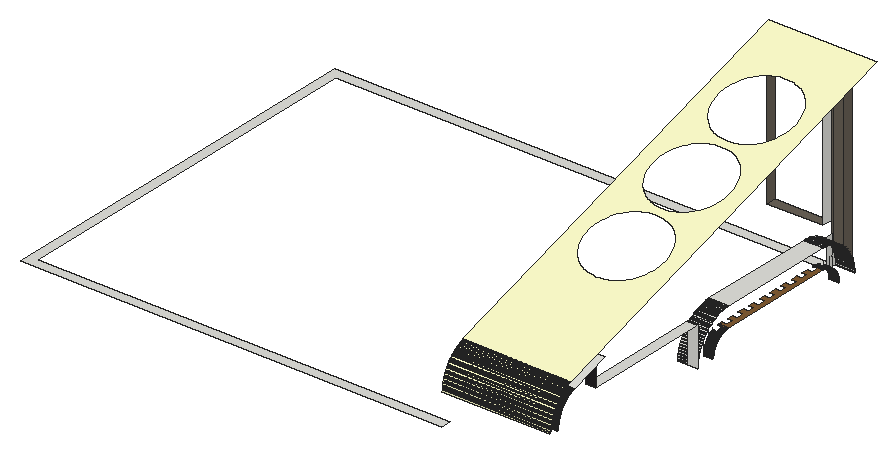
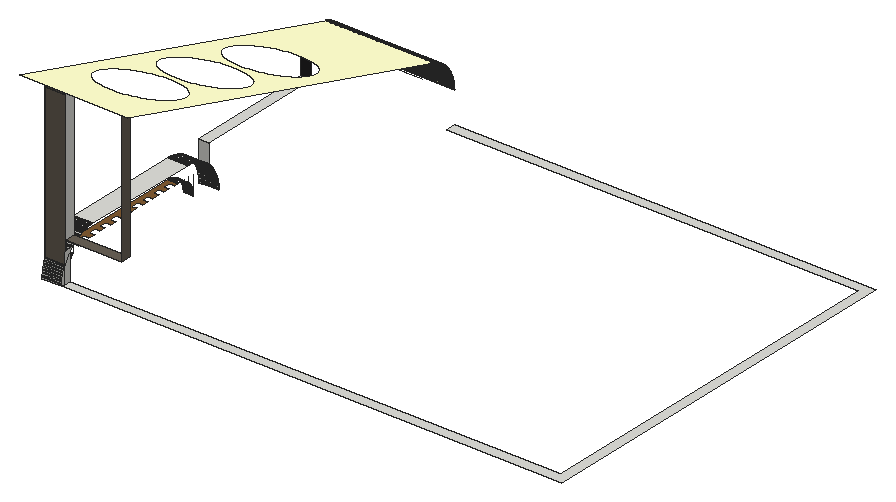
# SketchUp Ruby script. Lengths in inches.
U = 1.inch
M = Sketchup.active_model
def pt(a) = Geom::Point3d.new(a.map { |v| v * U })
def face(e, loops, mat)
  f = e.add_face(loops[0].map { |a| pt(a) })
  loops[1..].each { |l| e.add_face(l.map { |a| pt(a) }).erase! }
  f.material = f.back_material = mat if mat
  f
end
# faces: each face lists its corners as indices into pts; further lists are holes
def faces(e, pts, list, mat = nil) = list.each { |f| face(e, (f[0].is_a?(Array) ? f : [f]).map { |l| l.map { |i| pts[i] } }, mat) }
# xy, xz, yz: faces in a plane at the given z, y or x. An outline is a flat list of corners, or four numbers for a rectangle; further outlines are holes
def ring(l) = l.size == 4 ? [[l[0], l[1]], [l[2], l[1]], [l[2], l[3]], [l[0], l[3]]] : l.each_slice(2).to_a
def flat(e, list, mat, &to3) = list.each { |f| face(e, (f[0].is_a?(Array) ? f : [f]).map { |l| ring(l).map { |u, v| to3.(u, v) } }, mat) }
def xy(e, z, list, mat = nil) = flat(e, list, mat) { |x, y| [x, y, z] }
def xz(e, y, list, mat = nil) = flat(e, list, mat) { |x, z| [x, y, z] }
def yz(e, x, list, mat = nil) = flat(e, list, mat) { |y, z| [x, y, z] }
def lines(e, pts, list) = list.each { |a, b| e.add_line(pt(pts[a]), pt(pts[b])) }
# prism: a flat outline (further loops are holes) pulled along v
def prism(e, loops, v, mat = nil)
  f = face(e, loops, mat); d = Geom::Vector3d.new(v.map { |x| x * U })
  f.pushpull(f.normal.samedirection?(d) ? d.length : -d.length)
end
def box(e, o, s, mat = nil) = prism(e, [[o, [o[0] + s[0], o[1], o[2]], [o[0] + s[0], o[1] + s[1], o[2]], [o[0], o[1] + s[1], o[2]]]], [0, 0, s[2]], mat)
def at(x, y, z, deg = 0) = Geom::Transformation.translation(pt([x, y, z])) * Geom::Transformation.rotation(ORIGIN, Z_AXIS, deg.degrees)
def axes(o, x, y, z) = Geom::Transformation.new([*x, 0, *y, 0, *z, 0, *pt(o).to_a, 1])
def part(name) = M.definitions.add(name)
# library, detail: a bought-in or finely detailed component or shape, given as its bounding box
def library(name, o, s) = part(name).tap { |d| box(d.entities, o, s) }
def detail(e, o, s) = box(e.add_group.entities, o, s)
def put(e, d, t, mat = nil) = e.add_instance(d, t).tap { |i| i.material = mat if mat }
def group(e, t, mat = nil) = e.add_group.tap { |g| g.transformation = t; g.material = mat if mat }.entities
root = M.entities
M.materials.add("C08_Toffee_Ember").color = [130, 92, 50]
M.materials.add("E01_Mint_Frost").color = [255, 255, 204]
M.materials.add("Marble_07_1K").color = [36, 34, 36]
M.materials.add("Plaster_04_1K").color = [106, 98, 87]
xy(root,396,[[5.5,15,263.5,15,263.5,21,11.5,21,11.5,249,311.5,249,311.5,255,5.5,255]])
xy(root,408,[[317.5,159,317.5,161.32,320.5,161.32,320.5,165.4,317.5,165.4,317.5,169.49,320.5,169.49,320.5,173.57,317.5,173.57,317.5,177.66,320.5,177.66,320.5,181.74,317.5,181.74,317.5,185.82,320.5,185.82,320.5,189.91,317.5,189.91,317.5,193.99,320.5,193.99,320.5,198.08,317.5,198.08,317.5,202.16,320.5,202.16,320.5,206.24,317.5,206.24,317.5,210.33,320.5,210.33,320.5,214.41,317.5,214.41,317.5,218.5,320.5,218.5,320.5,222.58,317.5,222.58,317.5,226.66,320.5,226.66,320.5,230.75,317.5,230.75,317.5,231,323.5,231,323.5,159],[317.5,231,323.5,231.38]],"C08_Toffee_Ember")
xy(root,420,[[317.5,57,323.5,135],[311.5,159,323.5,231]])
xy(root,421,[[276.5,247,310.5,253]],"Plaster_04_1K")
xz(root,20.99,[[323.5,414.47,329.5,414.95]])
xz(root,57,[[317.5,420,323.5,437.47]],"Marble_07_1K")
xz(root,135,[[317.5,396,323.5,420]])
xz(root,243,[[317.5,396,323.5,396.38]],"C08_Toffee_Ember")
xz(root,247,[[317.5,413.98,323.5,498]],"Plaster_04_1K")
xz(root,253,[[311.5,406.93,323.5,500.01]],"Plaster_04_1K")
yz(root,276.5,[[247,421,253,503]],"Plaster_04_1K")
yz(root,310.5,[[247,421,253,503]])
yz(root,311.5,[[249,396,249,411.97,249.05,411.92,249.54,411.34,250.01,410.75,250.47,410.15,250.9,409.53,251.3125,408.9,251.71,408.25,251.85,408,252.08,407.6,252.43,406.93,252.76,406.25,253,405.72,253,396],[253,396,253,405.72,253.07,405.56,253.36,404.86,253.62,404.15,253.86,403.4375,254.08,402.71,254.28,401.98,254.45,401.25,254.6,400.51,254.73,399.76,254.83,399.01,254.91,398.26,254.96,397.51,254.99,396.76,255,396],[253,405.72,253,413.98,247,413.98,247.48,413.54,248.02,413.02,248.54,412.48,249,411.97,249.05,411.92,249.54,411.34,250.01,410.75,250.47,410.15,250.9,409.53,251.3125,408.9,251.71,408.25,251.85,408,252.08,407.6,252.43,406.93,252.76,406.25]])
yz(root,323.5,[[21,414,21,415.2,20.99,414.95,20.99,414.47]])
yz(root,323.5,[[252.43,406.93,253,406.93,253,500.01,247,498.15,247,413.98,247.48,413.54,248.02,413.02,248.54,412.48,249.05,411.92,249.54,411.34,250.01,410.75,250.47,410.15,250.9,409.53,251.3125,408.9,251.71,408.25,251.85,408,252.08,407.6]],"Plaster_04_1K")
p = [[317.5,135,396],[323.5,135,396],[323.5,135.03,396.75],[311.5,135.03,396.75],[311.5,135,396],[317.5,147,396],
  [317.5,147.01,396.375],[323.5,147.01,396.375],[323.5,147,396],[311.5,254.99,396.76],[323.5,254.99,396.76],[323.5,255,396],
  [311.5,255,396],[317.5,147.03,396.75],[323.5,147.03,396.75],[317.5,242.98,396.76],[317.5,243,396.38],[323.5,243,396.38],
  [323.5,242.98,396.76],[323.5,135.08,397.5],[311.5,135.08,397.5],[317.5,147.07,397.125],[323.5,147.07,397.125],[317.5,242.96,397.13],
  [323.5,242.96,397.13],[311.5,254.96,397.51],[323.5,254.96,397.51],[317.5,147.11,397.5],[323.5,147.11,397.5],[317.5,242.92,397.51],
  [323.5,242.92,397.51],[323.5,135.15,398.24],[311.5,135.15,398.24],[317.5,147.17,397.87],[323.5,147.17,397.87],[317.5,242.87,397.88],
  [323.5,242.87,397.88],[311.5,254.91,398.26],[323.5,254.91,398.26],[317.5,147.24,398.24],[323.5,147.24,398.24],[317.5,242.81,398.26],
  [323.5,242.81,398.26],[323.5,135.24,398.99],[311.5,135.24,398.99],[317.5,147.32,398.61],[323.5,147.32,398.61],[317.5,242.74,398.63],
  [323.5,242.74,398.63],[311.5,254.83,399.01],[323.5,254.83,399.01],[317.5,147.41,398.97],[323.5,147.41,398.97],[317.5,242.65,399],
  [323.5,242.65,399],[323.5,135.36,399.73],[311.5,135.36,399.73],[317.5,147.51,399.33],[323.5,147.51,399.33],[317.5,242.55,399.36],
  [323.5,242.55,399.36],[311.5,254.73,399.76],[323.5,254.73,399.76],[317.5,147.625,399.6875],[323.5,147.625,399.6875],[317.5,242.45,399.72],
  [323.5,242.45,399.72],[323.5,135.5,400.47],[311.5,135.5,400.47],[317.5,147.75,400.04],[323.5,147.75,400.04],[317.5,242.33,400.08],
  [323.5,242.33,400.08],[311.5,254.6,400.51],[323.5,254.6,400.51],[317.5,147.88,400.39],[323.5,147.88,400.39],[317.5,242.19,400.4375],
  [323.5,242.19,400.4375],[317.5,148.03,400.74],[323.5,148.03,400.74],[317.5,242.05,400.79],[323.5,242.05,400.79],[323.5,135.66,401.2],
  [311.5,135.66,401.2],[311.5,254.45,401.25],[323.5,254.45,401.25],[317.5,148.1875,401.08],[323.5,148.1875,401.08],[317.5,241.9,401.13],
  [323.5,241.9,401.13],[317.5,148.35,401.42],[323.5,148.35,401.42],[317.5,241.73,401.47],[323.5,241.73,401.47],[323.5,135.85,401.92],
  [311.5,135.85,401.92],[311.5,254.28,401.98],[323.5,254.28,401.98],[317.5,148.53,401.75],[323.5,148.53,401.75],[317.5,241.56,401.81],
  [323.5,241.56,401.81],[317.5,148.72,402.07],[323.5,148.72,402.07],[317.5,241.37,402.14],[323.5,241.37,402.14],[323.5,136.06,402.65],
  [311.5,136.06,402.65],[311.5,254.08,402.71],[323.5,254.08,402.71],[317.5,148.92,402.39],[323.5,148.92,402.39],[317.5,241.17,402.46],
  [323.5,241.17,402.46],[317.5,149.12,402.71],[323.5,149.12,402.71],[317.5,240.97,402.78],[323.5,240.97,402.78],[323.5,136.29,403.36],
  [311.5,136.29,403.36],[317.5,149.34,403.01],[323.5,149.34,403.01],[311.5,253.86,403.4375],[323.5,253.86,403.4375],[317.5,240.75,403.09],
  [323.5,240.75,403.09],[317.5,149.57,403.3125],[323.5,149.57,403.3125],[317.5,240.52,403.39],[323.5,240.52,403.39],[317.5,149.8,403.61],
  [323.5,149.8,403.61],[323.5,136.54,404.07],[311.5,136.54,404.07],[317.5,240.29,403.6875],[323.5,240.29,403.6875],[311.5,253.62,404.15],
  [323.5,253.62,404.15],[317.5,150.05,403.89],[323.5,150.05,403.89],[317.5,240.04,403.97],[323.5,240.04,403.97],[317.5,150.3,404.17],
  [323.5,150.3,404.17],[317.5,239.79,404.25],[323.5,239.79,404.25],[323.5,136.81,404.76],[311.5,136.81,404.76],[317.5,150.56,404.44],
  [323.5,150.56,404.44],[311.5,253.36,404.86],[323.5,253.36,404.86],[317.5,239.53,404.53],[323.5,239.53,404.53],[317.5,150.58,404.46],
  [317.5,150.83,404.7],[323.5,150.83,404.7],[317.5,239.25,404.79],[323.5,239.25,404.79],[317.5,151.11,404.95],[323.5,151.11,404.95],
  [323.5,137.1,405.45],[311.5,137.1,405.45],[317.5,238.97,405.04],[323.5,238.97,405.04],[311.5,253.07,405.56],[323.5,253.07,405.56],
  [317.5,151.39,405.2],[323.5,151.39,405.2],[323.5,238.6875,405.29],[320.5,238.6875,405.29],[320.5,238.92,405.09],[317.5,238.92,405.09],
  [317.5,151.6875,405.43],[323.5,151.6875,405.43],[323.5,238.39,405.52],[320.5,238.39,405.52],[317.5,151.99,405.66],[323.5,151.99,405.66],
  [323.5,137.42,406.14],[311.5,137.42,406.14],[323.5,238.09,405.75],[320.5,238.09,405.75],[311.5,252.76,406.25],[323.5,252.76,406.25],
  [311.5,253,405.72],[317.5,152.29,405.88],[323.5,152.29,405.88],[323.5,237.78,405.97],[320.5,237.78,405.97],[317.5,152.61,406.08],
  [323.5,152.61,406.08],[323.5,237.46,406.17],[320.5,237.46,406.17],[323.5,137.75,406.81],[311.5,137.75,406.81],[317.5,152.93,406.28],
  [323.5,152.93,406.28],[323.5,237.14,406.37],[320.5,237.14,406.37],[311.5,252.43,406.93],[323.5,252.43,406.93],[317.5,153.25,406.47],
  [323.5,153.25,406.47],[323.5,236.81,406.56],[320.5,236.81,406.56],[317.5,153.58,406.65],[323.5,153.58,406.65],[317.5,153.92,406.8125],
  [323.5,153.92,406.8125],[323.5,236.47,406.73],[320.5,236.47,406.73],[323.5,236.13,406.9],[320.5,236.13,406.9],[323.5,138.11,407.47],
  [311.5,138.11,407.47],[317.5,154.16,406.92],[320.5,154.16,406.92],[320.5,154.26,406.97],[323.5,154.26,406.97],[323.5,235.79,407.05],
  [320.5,235.79,407.05],[311.5,252.08,407.6],[323.5,252.08,407.6],[320.5,154.61,407.12],[323.5,154.61,407.12],[320.5,154.96,407.25],
  [323.5,154.96,407.25],[323.5,235.4375,407.19],[320.5,235.4375,407.19],[323.5,235.08,407.33],[320.5,235.08,407.33],[320.5,155.3125,407.375],
  [323.5,155.3125,407.375],[317.5,234.72,407.45],[317.5,234.83,407.41],[320.5,234.83,407.41],[323.5,234.72,407.45],[320.5,155.67,407.49],
  [323.5,155.67,407.49],[317.5,234.36,407.55],[323.5,234.36,407.55],[323.5,138.48,408.11],[311.5,138.48,408.11],[320.5,156.03,407.59],
  [323.5,156.03,407.59],[320.5,156.39,407.68],[323.5,156.39,407.68],[317.5,234,407.65],[323.5,234,407.65],[311.5,251.85,408],
  [323.5,251.85,408],[320.5,156.76,407.76],[323.5,156.76,407.76],[317.5,233.26,407.81],[317.5,233.63,407.74],[323.5,233.63,407.74],
  [323.5,233.26,407.81],[320.5,157.13,407.83],[323.5,157.13,407.83],[320.5,157.5,407.89],[323.5,157.5,407.89],[317.5,232.88,407.87],
  [323.5,232.88,407.87],[320.5,157.74,407.92],[317.5,157.74,407.92],[317.5,157.875,407.93],[323.5,157.875,407.93],[317.5,158.25,407.97],
  [323.5,158.25,407.97],[317.5,232.13,407.96],[317.5,232.51,407.92],[323.5,232.51,407.92],[323.5,232.13,407.96],[317.5,158.625,407.99],
  [323.5,158.625,407.99],[317.5,159,408],[323.5,159,408],[317.5,231.38,408],[317.5,231.76,407.98],[323.5,231.76,407.98],
  [323.5,231.38,408],[311.5,251.71,408.25],[323.5,251.71,408.25],[323.5,138.88,408.75],[311.5,138.88,408.75],[311.5,251.3125,408.9],
  [323.5,251.3125,408.9],[323.5,139.3,409.375],[311.5,139.3,409.375],[311.5,250.9,409.53],[323.5,250.9,409.53],[323.5,139.73,409.99],
  [311.5,139.73,409.99],[311.5,250.47,410.15],[323.5,250.47,410.15],[323.5,140.18,410.59],[311.5,140.18,410.59],[311.5,250.01,410.75],
  [323.5,250.01,410.75],[323.5,140.65,411.17],[311.5,140.65,411.17],[311.5,249.54,411.34],[323.5,249.54,411.34],[323.5,141.14,411.74],
  [311.5,141.14,411.74],[311.5,141,411.58],[311.5,249.05,411.92],[323.5,249.05,411.92],[323.5,141.65,412.29],[311.5,141.65,412.29],
  [311.5,248.54,412.48],[323.5,248.54,412.48],[311.5,249,411.97],[323.5,142.17,412.83],[311.5,142.17,412.83],[311.5,248.02,413.02],
  [323.5,248.02,413.02],[323.5,142.71,413.35],[311.5,142.71,413.35],[311.5,247.48,413.54],[323.5,247.48,413.54],[323.5,143.26,413.86],
  [311.5,143.26,413.86],[311.5,247,413.98],[317.5,247,413.98],[323.5,247,413.98],[323.5,143.83,414.35],[311.5,143.83,414.35],
  [323.5,21,414],[323.5,20.99,414.47],[329.5,20.99,414.47],[329.5,21,414],[323.5,246.92,414.05],[311.5,246.92,414.05],
  [311.5,246.34,414.54],[323.5,246.34,414.54],[323.5,144.41,414.82],[311.5,144.41,414.82],[311.5,245.75,415.01],[323.5,245.75,415.01],
  [323.5,145.01,415.27],[311.5,145.01,415.27],[323.5,20.99,414.95],[323.5,21,415.2],[329.5,21,415.2],[329.5,20.99,414.95],
  [311.5,245.15,415.47],[323.5,245.15,415.47],[323.5,21.01,415.42],[329.5,21.01,415.42],[263.5,15,415.29],[329.5,15,415.29],
  [329.5,15.02,415.87],[263.5,15.02,415.87],[323.5,145.625,415.7],[311.5,145.625,415.7],[323.5,21.03,415.9],[329.5,21.03,415.9],
  [311.5,244.53,415.9],[323.5,244.53,415.9],[323.5,146.25,416.12],[311.5,146.25,416.12],[329.5,15.0625,416.5],[263.5,15.0625,416.5],
  [323.5,21.07,416.37],[329.5,21.07,416.37],[311.5,243.9,416.3125],[323.5,243.9,416.3125],[323.5,146.89,416.52],[311.5,146.89,416.52],
  [311.5,243.25,416.71],[323.5,243.25,416.71],[323.5,21.125,416.84],[329.5,21.125,416.84],[329.5,15.12,417.12],[263.5,15.12,417.12],
  [323.5,147.53,416.89],[311.5,147.53,416.89],[311.5,242.6,417.08],[323.5,242.6,417.08],[323.5,21.19,417.31],[329.5,21.19,417.31],
  [323.5,148.19,417.25],[311.5,148.19,417.25],[329.5,15.19,417.74],[263.5,15.19,417.74],[311.5,241.93,417.43],[323.5,241.93,417.43],
  [323.5,148.86,417.58],[311.5,148.86,417.58],[323.5,21.27,417.78],[329.5,21.27,417.78],[311.5,241.25,417.76],[323.5,241.25,417.76],
  [323.5,149.55,417.9],[311.5,149.55,417.9],[329.5,15.28,418.36],[263.5,15.28,418.36],[323.5,21.36,418.24],[329.5,21.36,418.24],
  [311.5,240.56,418.07],[323.5,240.56,418.07],[323.5,150.24,418.19],[311.5,150.24,418.19],[311.5,239.86,418.36],[323.5,239.86,418.36],
  [323.5,21.46,418.71],[329.5,21.46,418.71],[323.5,150.93,418.46],[311.5,150.93,418.46],[329.5,15.39,418.97],[263.5,15.39,418.97],
  [311.5,239.15,418.62],[323.5,239.15,418.62],[311.5,239.59,418.46],[323.5,151.64,418.71],[311.5,151.64,418.71],[311.5,238.4375,418.86],
  [323.5,238.4375,418.86],[323.5,21.57,419.17],[329.5,21.57,419.17],[323.5,152.35,418.94],[311.5,152.35,418.94],[323.5,153.08,419.15],
  [311.5,153.08,419.15],[311.5,237.71,419.08],[323.5,237.71,419.08],[329.5,15.51,419.58],[263.5,15.51,419.58],[311.5,236.98,419.28],
  [323.5,236.98,419.28],[323.5,21.7,419.625],[329.5,21.7,419.625],[323.5,153.8,419.34],[311.5,153.8,419.34],[323.5,154.53,419.5],
  [311.5,154.53,419.5],[311.5,236.25,419.45],[323.5,236.25,419.45],[323.5,155.27,419.64],[311.5,155.27,419.64],[311.5,235.51,419.6],
  [323.5,235.51,419.6],[329.5,15.65,420.19],[263.5,15.65,420.19],[323.5,21.84,420.08],[329.5,21.84,420.08],[323.5,156.01,419.76],
  [311.5,156.01,419.76],[311.5,234.76,419.73],[323.5,234.76,419.73],[311.5,234.01,419.83],[323.5,234.01,419.83],[323.5,156.76,419.85],
  [311.5,156.76,419.85],[311.5,233.26,419.91],[323.5,233.26,419.91],[323.5,157.5,419.92],[311.5,157.5,419.92],[323.5,158.25,419.97],
  [311.5,158.25,419.97],[311.5,232.51,419.96],[323.5,232.51,419.96],[323.5,159,420],[311.5,159,420],[311.5,231,420],
  [323.5,231,420],[323.5,231.76,419.99],[311.5,231.76,419.99],[323.5,21.99,420.53],[329.5,21.99,420.53],[329.5,15.81,420.8],
  [263.5,15.81,420.8],[323.5,22.15,420.97],[329.5,22.15,420.97],[329.5,15.98,421.4],[263.5,15.98,421.4],[323.5,22.32,421.41],
  [329.5,22.32,421.41],[329.5,16.16,421.99],[263.5,16.16,421.99],[323.5,22.51,421.85],[329.5,22.51,421.85],[323.5,22.7,422.28],
  [329.5,22.7,422.28],[329.5,16.37,422.58],[263.5,16.37,422.58],[323.5,22.91,422.71],[329.5,22.91,422.71],[329.5,16.58,423.17],
  [263.5,16.58,423.17],[323.5,23.13,423.13],[329.5,23.13,423.13],[323.5,23.36,423.54],[329.5,23.36,423.54],[329.5,16.82,423.75],
  [263.5,16.82,423.75],[323.5,23.6,423.95],[329.5,23.6,423.95],[329.5,17.07,424.32],[263.5,17.07,424.32],[323.5,23.85,424.35],
  [329.5,23.85,424.35],[329.5,17.33,424.89],[263.5,17.33,424.89],[323.5,24.11,424.75],[329.5,24.11,424.75],[323.5,24.39,425.14],
  [329.5,24.39,425.14],[329.5,17.61,425.44],[263.5,17.61,425.44],[323.5,24.67,425.52],[329.5,24.67,425.52],[329.5,17.9,426],
  [263.5,17.9,426],[323.5,24.96,425.89],[329.5,24.96,425.89],[323.5,25.26,426.26],[329.5,25.26,426.26],[329.5,18.21,426.54],
  [263.5,18.21,426.54],[323.5,25.58,426.61],[329.5,25.58,426.61],[329.5,18.53,427.07],[263.5,18.53,427.07],[323.5,25.9,426.96],
  [329.5,25.9,426.96],[323.5,26.23,427.3],[329.5,26.23,427.3],[329.5,18.87,427.6],[263.5,18.87,427.6],[323.5,26.57,427.64],
  [329.5,26.57,427.64],[329.5,19.22,428.12],[263.5,19.22,428.12],[323.5,26.91,427.96],[329.5,26.91,427.96],[323.5,27.27,428.27],
  [329.5,27.27,428.27],[329.5,19.58,428.625],[263.5,19.58,428.625],[323.5,27.63,428.58],[329.5,27.63,428.58],[329.5,19.96,429.12],
  [263.5,19.96,429.12],[323.5,28.01,428.87],[329.5,28.01,428.87],[323.5,28.39,429.15],[329.5,28.39,429.15],[329.5,20.35,429.61],
  [263.5,20.35,429.61],[323.5,28.77,429.43],[329.5,28.77,429.43],[323.5,29.17,429.69],[329.5,29.17,429.69],[329.5,20.75,430.09],
  [263.5,20.75,430.09],[323.5,29.57,429.94],[329.5,29.57,429.94],[323.5,29.98,430.1875],[329.5,29.98,430.1875],[329.5,21.17,430.55],
  [263.5,21.17,430.55],[263.5,21,430.37],[323.5,30.39,430.42],[329.5,30.39,430.42],[323.5,30.81,430.64],[329.5,30.81,430.64],
  [329.5,21.59,431.01],[263.5,21.59,431.01],[323.5,31.23,430.85],[329.5,31.23,430.85],[323.5,31.67,431.05],[329.5,31.67,431.05],
  [329.5,22.03,431.45],[263.5,22.03,431.45],[323.5,32.1,431.23],[329.5,32.1,431.23],[323.5,32.54,431.41],[329.5,32.54,431.41],
  [323.5,32.99,431.57],[329.5,32.99,431.57],[329.5,22.49,431.88],[263.5,22.49,431.88],[323.5,33.4375,431.72],[329.5,33.4375,431.72],
  [323.5,57,439.04],[329.5,57,439.04],[323.5,38,433.14],[323.5,39,433.45],[323.5,40,433.76],[329.5,22.95,432.3],
  [263.5,22.95,432.3],[263.5,22.61,432],[329.5,23.42,432.71],[263.5,23.42,432.71],[329.5,23.9,433.1],[263.5,23.9,433.1],
  [329.5,24.4,433.49],[263.5,24.4,433.49],[329.5,24.9,433.85],[263.5,24.9,433.85],[329.5,25.42,434.21],[263.5,25.42,434.21],
  [329.5,25.9375,434.55],[263.5,25.9375,434.55],[329.5,26.47,434.88],[263.5,26.47,434.88],[329.5,27.01,435.19],[263.5,27.01,435.19],
  [329.5,27.56,435.49],[263.5,27.56,435.49],[329.5,28.12,435.77],[263.5,28.12,435.77],[329.5,28.68,436.04],[263.5,28.68,436.04],
  [329.5,29.25,436.3],[263.5,29.25,436.3],[329.5,29.83,436.54],[263.5,29.83,436.54],[329.5,30.41,436.76],[263.5,30.41,436.76],
  [329.5,30.96,436.95],[263.5,30.96,436.95],[329.5,264.19,509.34],[263.5,264.19,509.34],[263.5,247,504],[294.99,137.32,469.96],
  [296.5,137.37,469.98],[298.01,137.32,469.96],[299.51,137.1875,469.92],[301,136.96,469.85],[302.47,136.65,469.75],[303.92,136.24,469.63],
  [305.33,135.76,469.48],[306.72,135.18,469.3],[308.0625,134.53,469.1],[309.36,133.8,468.87],[310.61,132.99,468.62],[311.8,132.11,468.34],
  [312.93,131.15,468.05],[314,130.14,467.73],[314.99,129.06,467.4],[315.92,127.92,467.04],[316.76,126.73,466.67],[317.53,125.49,466.29],
  [318.22,124.2,465.89],[318.81,122.88,465.48],[319.33,121.53,465.06],[319.75,120.15,464.63],[320.07,118.74,464.2],[320.3125,117.32,463.75],
  [320.45,115.88,463.31],[320.5,114.44,462.86],[320.45,113.01,462.42],[320.3125,111.57,461.97],[320.07,110.15,461.53],[319.75,108.74,461.09],
  [319.33,107.36,460.66],[318.81,106.01,460.24],[318.22,104.69,459.83],[317.53,103.4,459.44],[316.76,102.16,459.05],[315.92,100.97,458.68],
  [314.99,99.83,458.33],[314,98.75,457.99],[312.93,97.74,457.68],[311.8,96.78,457.38],[310.61,95.9,457.11],[309.36,95.09,456.86],
  [308.0625,94.36,456.63],[306.72,93.7,456.43],[305.33,93.13,456.25],[303.92,92.65,456.1],[302.47,92.24,455.97],[301,91.93,455.875],
  [299.51,91.7,455.8],[298.01,91.57,455.76],[297.99,91.57,455.76],[296.5,91.52,455.75],[295.01,91.57,455.76],[294.99,91.57,455.76],
  [293.49,91.7,455.8],[292,91.93,455.875],[290.53,92.24,455.97],[289.08,92.65,456.1],[287.67,93.13,456.25],[286.28,93.7,456.43],
  [284.9375,94.36,456.63],[283.64,95.09,456.86],[282.39,95.9,457.11],[281.2,96.78,457.38],[280.07,97.74,457.68],[279,98.75,457.99],
  [278.01,99.83,458.33],[277.08,100.97,458.68],[276.24,102.16,459.05],[275.47,103.4,459.44],[274.78,104.69,459.83],[274.19,106.01,460.24],
  [273.67,107.36,460.66],[273.25,108.74,461.09],[272.93,110.15,461.53],[272.6875,111.57,461.97],[272.55,113.01,462.42],[272.5,114.44,462.86],
  [272.55,115.88,463.31],[272.6875,117.32,463.75],[272.93,118.74,464.2],[273.25,120.15,464.63],[273.67,121.53,465.06],[274.19,122.88,465.48],
  [274.78,124.2,465.89],[275.47,125.49,466.29],[276.24,126.73,466.67],[277.08,127.92,467.04],[278.01,129.06,467.4],[279,130.14,467.73],
  [280.07,131.15,468.05],[281.2,132.11,468.34],[282.39,132.99,468.62],[283.64,133.8,468.87],[284.9375,134.53,469.1],[286.28,135.18,469.3],
  [287.67,135.76,469.48],[289.08,136.24,469.63],[290.53,136.65,469.75],[292,136.96,469.85],[293.49,137.1875,469.92],[296.85,190.96,486.61],
  [296.5,190.95,486.61],[296.15,190.96,486.61],[294.99,191,486.62],[293.49,191.13,486.66],[292,191.36,486.73],[290.53,191.67,486.83],
  [289.08,192.07,486.95],[287.67,192.56,487.1],[286.28,193.13,487.28],[284.9375,193.79,487.49],[283.64,194.52,487.71],[282.39,195.33,487.96],
  [281.2,196.21,488.24],[280.07,197.16,488.53],[279,198.18,488.85],[278.01,199.26,489.18],[277.08,200.4,489.54],[276.24,201.59,489.91],
  [275.47,202.83,490.29],[274.78,204.11,490.69],[274.19,205.43,491.1],[273.67,206.79,491.52],[273.25,208.17,491.95],[272.93,209.58,492.39],
  [272.6875,211,492.83],[272.55,212.43,493.27],[272.5,213.87,493.72],[272.55,215.3125,494.17],[272.6875,216.74,494.61],[272.93,218.17,495.05],
  [273.25,219.57,495.49],[273.67,220.96,495.92],[274.19,222.31,496.34],[274.78,223.63,496.75],[275.47,224.91,497.15],[276.24,226.15,497.53],
  [277.08,227.35,497.9],[278.01,228.48,498.25],[279,229.5625,498.59],[280.07,230.58,498.9],[281.2,231.53,499.2],[282.39,232.42,499.47],
  [283.64,233.23,499.73],[284.9375,233.96,499.95],[286.28,234.61,500.16],[287.67,235.18,500.33],[289.08,235.67,500.48],[290.53,236.07,500.61],
  [292,236.39,500.71],[293.49,236.61,500.78],[294.99,236.75,500.82],[296.15,236.78,500.83],[296.5,236.79,500.83],[296.85,236.78,500.83],
  [298.01,236.75,500.82],[299.51,236.61,500.78],[301,236.39,500.71],[302.47,236.07,500.61],[303.92,235.67,500.48],[305.33,235.18,500.33],
  [306.72,234.61,500.16],[308.0625,233.96,499.95],[309.36,233.23,499.73],[310.61,232.42,499.47],[311.8,231.53,499.2],[312.93,230.58,498.9],
  [314,229.5625,498.59],[314.99,228.48,498.25],[315.92,227.35,497.9],[316.76,226.15,497.53],[317.53,224.91,497.15],[318.22,223.63,496.75],
  [318.81,222.31,496.34],[319.33,220.96,495.92],[319.75,219.57,495.49],[320.07,218.17,495.05],[320.3125,216.74,494.61],[320.45,215.3125,494.17],
  [320.5,213.87,493.72],[320.45,212.43,493.27],[320.3125,211,492.83],[320.07,209.58,492.39],[319.75,208.17,491.95],[319.33,206.79,491.52],
  [318.81,205.43,491.1],[318.22,204.11,490.69],[317.53,202.83,490.29],[316.76,201.59,489.91],[315.92,200.4,489.54],[314.99,199.26,489.18],
  [314,198.18,488.85],[312.93,197.16,488.53],[311.8,196.21,488.24],[310.61,195.33,487.96],[309.36,194.52,487.71],[308.0625,193.79,487.49],
  [306.72,193.13,487.28],[305.33,192.56,487.1],[303.92,192.07,486.95],[302.47,191.67,486.83],[301,191.36,486.73],[299.51,191.13,486.66],
  [298.01,191,486.62],[298.01,141.45,471.24],[296.5,141.4,471.23],[294.99,141.45,471.24],[293.49,141.58,471.28],[292,141.81,471.35],
  [290.53,142.12,471.45],[289.08,142.52,471.58],[287.67,143.01,471.73],[286.28,143.58,471.91],[284.9375,144.24,472.11],[283.64,144.97,472.34],
  [282.39,145.78,472.59],[281.2,146.66,472.86],[280.07,147.61,473.16],[279,148.63,473.47],[278.01,149.71,473.81],[277.08,150.85,474.16],
  [276.24,152.04,474.53],[275.47,153.28,474.91],[274.78,154.5625,475.3125],[274.19,155.88,475.72],[273.67,157.24,476.14],[273.25,158.62,476.57],
  [272.93,160.03,477.01],[272.6875,161.45,477.45],[272.55,162.88,477.89],[272.5,164.32,478.34],[272.55,165.76,478.79],[272.6875,167.2,479.23],
  [272.93,168.62,479.67],[273.25,170.02,480.11],[273.67,171.41,480.54],[274.19,172.76,480.96],[274.78,174.08,481.37],[275.47,175.37,481.77],
  [276.24,176.6,482.15],[277.08,177.8,482.52],[278.01,178.93,482.875],[279,180.01,483.21],[280.07,181.03,483.53],[281.2,181.98,483.82],
  [282.39,182.87,484.1],[283.64,183.68,484.35],[284.9375,184.41,484.58],[286.28,185.0625,484.78],[287.67,185.63,484.96],[289.08,186.12,485.11],
  [290.53,186.52,485.23],[292,186.84,485.33],[293.49,187.0625,485.4],[294.99,187.2,485.44],[295.05,187.2,485.44],[296.5,187.24,485.46],
  [297.95,187.2,485.44],[298.01,187.2,485.44],[299.51,187.0625,485.4],[301,186.84,485.33],[302.47,186.52,485.23],[303.92,186.12,485.11],
  [305.33,185.63,484.96],[306.72,185.0625,484.78],[308.0625,184.41,484.58],[309.36,183.68,484.35],[310.61,182.87,484.1],[311.8,181.98,483.82],
  [312.93,181.03,483.53],[314,180.01,483.21],[314.99,178.93,482.875],[315.92,177.8,482.52],[316.76,176.6,482.15],[317.53,175.37,481.77],
  [318.22,174.08,481.37],[318.81,172.76,480.96],[319.33,171.41,480.54],[319.75,170.02,480.11],[320.07,168.62,479.67],[320.3125,167.2,479.23],
  [320.45,165.76,478.79],[320.5,164.32,478.34],[320.45,162.88,477.89],[320.3125,161.45,477.45],[320.07,160.03,477.01],[319.75,158.62,476.57],
  [319.33,157.24,476.14],[318.81,155.88,475.72],[318.22,154.5625,475.3125],[317.53,153.28,474.91],[316.76,152.04,474.53],[315.92,150.85,474.16],
  [314.99,149.71,473.81],[314,148.63,473.47],[312.93,147.61,473.16],[311.8,146.66,472.86],[310.61,145.78,472.59],[309.36,144.97,472.34],
  [308.0625,144.24,472.11],[306.72,143.58,471.91],[305.33,143.01,471.73],[303.92,142.52,471.58],[302.47,142.12,471.45],[301,141.81,471.35],
  [299.51,141.58,471.28],[317.5,39.83,432],[317.5,57,432],[263.5,39.83,432],[317.5,57,437.47],[317.5,234.83,408],
  [317.5,238.92,408],[317.5,243,396],[317.5,243,408],[317.5,157.74,408],[317.5,154.16,408],[317.5,150.58,408],
  [317.5,147,408]]
faces(root,p,[[0,1,2,3,4],[9,10,11,12],[3,2,19,20],[25,26,10,9],[20,19,31,32],[37,38,26,25],[32,31,43,44],[49,50,38,37],
  [44,43,55,56],[61,62,50,49],[56,55,67,68],[73,74,62,61],[68,67,83,84],[85,86,74,73],[84,83,95,96],[97,98,86,85],
  [96,95,107,108],[109,110,98,97],[108,107,119,120],[123,124,110,109],[120,119,133,134],[137,138,124,123],[134,133,147,148],[151,152,138,137],
  [148,147,162,163],[166,167,152,151],[163,162,180,181],[184,185,167,166,186],[181,180,195,196],[201,202,185,184],[196,195,215,216],[223,224,202,201],
  [216,215,243,244],[251,252,224,223],[283,284,252,251],[244,243,285,286],[287,288,284,283],[286,285,289,290],[291,292,288,287],[290,289,293,294],
  [295,296,292,291],[294,293,297,298],[299,300,296,295],[298,297,301,302],[303,304,300,299],[302,301,305,306,307],[308,309,304,303],[306,305,310,311],
  [312,313,309,308,314],[311,310,315,316],[317,318,313,312],[316,315,319,320],[321,322,318,317],[320,319,323,324],[321,325,326,327,322],[324,323,328,329],
  [330,331,332,333],[334,327,326,325,335],[336,337,334,335],[329,328,338,339],[340,341,337,336],[339,338,342,343],[344,345,346,347],[348,349,341,340],
  [345,350,351,346],[343,342,356,357],[350,358,359,351],[360,361,349,348],[357,356,362,363],[358,366,367,359],[368,369,361,360],[363,362,370,371],
  [372,373,369,368],[366,374,375,367],[371,370,378,379],[380,381,373,372],[374,382,383,375],[379,378,384,385],[388,389,381,380],[385,384,390,391],
  [382,392,393,383],[394,395,389,388],[391,390,396,397],[392,400,401,393],[402,403,395,394],[397,396,404,405],[406,407,403,402],[400,408,409,401],
  [405,404,410,411],[414,415,407,406,416],[411,410,417,418],[419,420,415,414],[408,421,422,409],[418,417,423,424],[424,423,425,426],[427,428,420,419],
  [431,432,428,427],[421,433,434,422],[426,425,435,436],[436,435,437,438],[439,440,432,431],[438,437,441,442],[443,444,440,439],[433,447,448,434],
  [442,441,449,450],[451,452,444,443],[453,454,452,451],[450,449,455,456],[457,458,454,453],[456,455,459,460],[460,459,461,462],[463,464,458,457],
  [462,461,465,466],[467,468,469,470],[470,469,464,463],[447,471,472,448],[471,475,476,472],[475,479,480,476],[479,483,484,480],[483,485,486,484],
  [485,489,490,486],[489,493,494,490],[493,495,496,494],[495,499,500,496],[499,503,504,500],[503,507,508,504],[507,509,510,508],[509,513,514,510],
  [513,517,518,514],[517,519,520,518],[519,523,524,520],[523,527,528,524],[527,529,530,528],[529,533,534,530],[533,537,538,534],[537,539,540,538],
  [539,543,544,540],[543,547,548,544],[547,549,550,548],[549,553,554,550],[553,555,556,554],[555,559,560,556],[559,561,562,560],[561,566,567,562],
  [566,568,569,567],[568,572,573,569],[572,574,575,573],[574,578,579,575],[578,580,581,579],[580,582,583,581],[582,586,587,583],[588,589,587,586,590,591,592]])
faces(root,p,[[5,6,7,8],[6,13,14,7],[15,16,17,18],[13,21,22,14],[23,15,18,24],[21,27,28,22],[29,23,24,30],[27,33,34,28],
  [35,29,30,36],[33,39,40,34],[41,35,36,42],[39,45,46,40],[47,41,42,48],[45,51,52,46],[53,47,48,54],[51,57,58,52],
  [59,53,54,60],[57,63,64,58],[65,59,60,66],[63,69,70,64],[71,65,66,72],[69,75,76,70],[77,71,72,78],[75,79,80,76],
  [81,77,78,82],[79,87,88,80],[89,81,82,90],[87,91,92,88],[93,89,90,94],[91,99,100,92],[101,93,94,102],[99,103,104,100],
  [105,101,102,106],[103,111,112,104],[113,105,106,114],[111,115,116,112],[117,113,114,118],[115,121,122,116],[125,117,118,126],[121,127,128,122],
  [129,125,126,130],[127,131,132,128],[135,129,130,136],[131,139,140,132],[141,135,136,142],[139,143,144,140],[145,141,142,146],[143,149,150,144],
  [153,145,146,154],[149,155,156,157,150],[158,153,154,159],[156,160,161,157],[164,158,159,165],[160,168,169,161],[170,171,172,173,164,165],[168,174,175,169],
  [176,177,171,170],[174,178,179,175],[182,183,177,176],[178,187,188,179],[189,190,183,182],[187,191,192,188],[193,194,190,189],[191,197,198,192],
  [199,200,194,193],[197,203,204,198],[205,206,200,199],[203,207,208,204],[207,209,210,208],[211,212,206,205],[213,214,212,211],[209,217,218,219,220,210],
  [221,222,214,213],[220,219,225,226],[226,225,227,228],[229,230,222,221],[231,232,230,229],[228,227,233,234],[235,236,237,232,231,238],[234,233,239,240],
  [241,235,238,242],[240,239,245,246],[246,245,247,248],[249,241,242,250],[248,247,253,254],[255,256,257,258],[256,249,250,257],[254,253,259,260],
  [260,259,261,262],[263,255,258,264],[262,261,265,266,267,268],[267,269,270,268],[271,272,273,274],[272,263,264,273],[269,275,276,270],[275,277,278,276],
  [279,280,281,282],[280,271,274,281]],"C08_Toffee_Ember")
faces(root,p,[[352,353,354,355],[355,354,364,365],[365,364,376,377],[377,376,386,387],[387,386,398,399],[399,398,412,413],[413,412,429,430],[430,429,445,446],
  [446,445,473,474],[474,473,477,478],[478,477,481,482],[482,481,487,488],[488,487,491,492],[492,491,497,498],[498,497,501,502],[502,501,505,506],
  [506,505,511,512],[512,511,515,516],[516,515,521,522],[522,521,525,526],[526,525,531,532],[532,531,535,536],[536,535,541,542],[542,541,545,546],
  [546,545,551,552],[552,551,557,558],[558,557,563,564,565],[564,563,570,571],[571,570,576,577],[577,576,584,585],[585,584,593,594,595],[594,593,596,597],
  [597,596,598,599],[599,598,600,601],[601,600,602,603],[603,602,604,605],[605,604,606,607],[607,606,608,609],[609,608,610,611],[611,610,612,613],
  [613,612,614,615],[615,614,616,617],[617,616,618,619],[619,618,620,621],[621,620,622,623],[623,622,624,625],[[625,624,626,627,628],[629,630,631,632,633,634,635,636,637,638,639,640,641,642,643,644,645,646,647,648,649,650,651,652,653,654,655,656,657,658,659,660,661,662,663,664,665,666,667,668,669,670,671,672,673,674,675,676,677,678,679,680,681,682,683,684,685,686,687,688,689,690,691,692,693,694,695,696,697,698,699,700,701,702,703,704,705,706,707,708,709,710,711,712,713,714,715,716,717,718,719,720,721,722,723,724,725,726,727,728,729,730],[731,732,733,734,735,736,737,738,739,740,741,742,743,744,745,746,747,748,749,750,751,752,753,754,755,756,757,758,759,760,761,762,763,764,765,766,767,768,769,770,771,772,773,774,775,776,777,778,779,780,781,782,783,784,785,786,787,788,789,790,791,792,793,794,795,796,797,798,799,800,801,802,803,804,805,806,807,808,809,810,811,812,813,814,815,816,817,818,819,820,821,822,823,824,825,826,827,828,829,830,831,832,833,834],[835,836,837,838,839,840,841,842,843,844,845,846,847,848,849,850,851,852,853,854,855,856,857,858,859,860,861,862,863,864,865,866,867,868,869,870,871,872,873,874,875,876,877,878,879,880,881,882,883,884,885,886,887,888,889,890,891,892,893,894,895,896,897,898,899,900,901,902,903,904,905,906,907,908,909,910,911,912,913,914,915,916,917,918,919,920,921,922,923,924,925,926,927,928,929,930,931,932,933,934,935,936]]],"E01_Mint_Frost")
lines(root,p,[[937,938],[937,939],[940,937],[236,941],[173,942],[943,944],[266,945],[217,946],[155,947],[5,948]])
